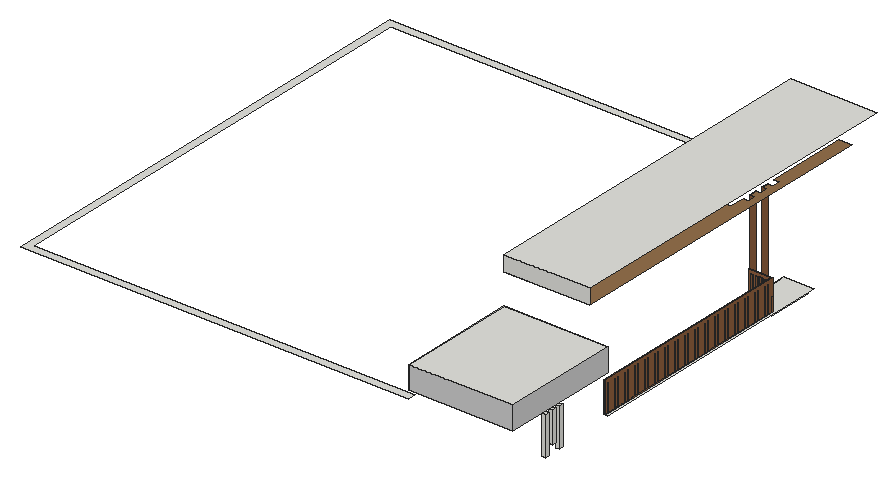
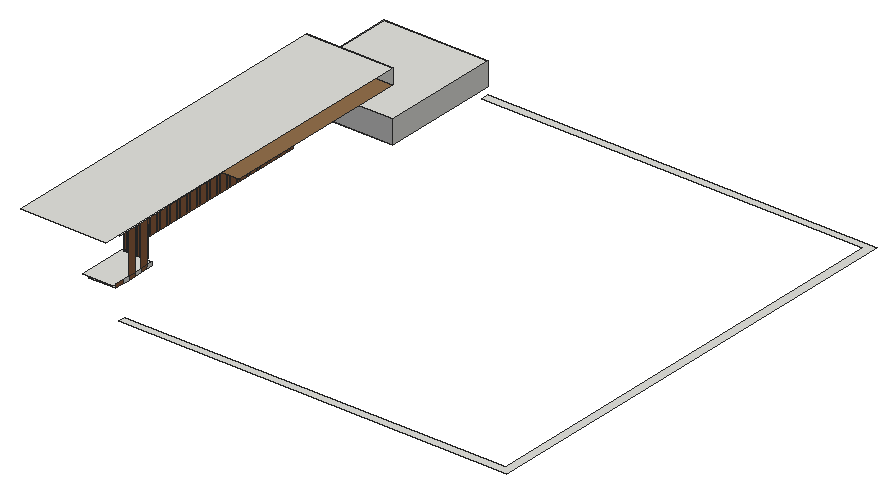
# SketchUp Ruby script. Lengths in inches.
U = 1.inch
M = Sketchup.active_model
def pt(a) = Geom::Point3d.new(a.map { |v| v * U })
def face(e, loops, mat)
  f = e.add_face(loops[0].map { |a| pt(a) })
  loops[1..].each { |l| e.add_face(l.map { |a| pt(a) }).erase! }
  f.material = f.back_material = mat if mat
  f
end
# faces: each face lists its corners as indices into pts; further lists are holes
def faces(e, pts, list, mat = nil) = list.each { |f| face(e, (f[0].is_a?(Array) ? f : [f]).map { |l| l.map { |i| pts[i] } }, mat) }
# xy, xz, yz: faces in a plane at the given z, y or x. An outline is a flat list of corners, or four numbers for a rectangle; further outlines are holes
def ring(l) = l.size == 4 ? [[l[0], l[1]], [l[2], l[1]], [l[2], l[3]], [l[0], l[3]]] : l.each_slice(2).to_a
def flat(e, list, mat, &to3) = list.each { |f| face(e, (f[0].is_a?(Array) ? f : [f]).map { |l| ring(l).map { |u, v| to3.(u, v) } }, mat) }
def xy(e, z, list, mat = nil) = flat(e, list, mat) { |x, y| [x, y, z] }
def xz(e, y, list, mat = nil) = flat(e, list, mat) { |x, z| [x, y, z] }
def yz(e, x, list, mat = nil) = flat(e, list, mat) { |y, z| [x, y, z] }
def lines(e, pts, list) = list.each { |a, b| e.add_line(pt(pts[a]), pt(pts[b])) }
# prism: a flat outline (further loops are holes) pulled along v
def prism(e, loops, v, mat = nil)
  f = face(e, loops, mat); d = Geom::Vector3d.new(v.map { |x| x * U })
  f.pushpull(f.normal.samedirection?(d) ? d.length : -d.length)
end
def box(e, o, s, mat = nil) = prism(e, [[o, [o[0] + s[0], o[1], o[2]], [o[0] + s[0], o[1] + s[1], o[2]], [o[0], o[1] + s[1], o[2]]]], [0, 0, s[2]], mat)
def at(x, y, z, deg = 0) = Geom::Transformation.translation(pt([x, y, z])) * Geom::Transformation.rotation(ORIGIN, Z_AXIS, deg.degrees)
def axes(o, x, y, z) = Geom::Transformation.new([*x, 0, *y, 0, *z, 0, *pt(o).to_a, 1])
def part(name) = M.definitions.add(name)
# library, detail: a bought-in or finely detailed component or shape, given as its bounding box
def library(name, o, s) = part(name).tap { |d| box(d.entities, o, s) }
def detail(e, o, s) = box(e.add_group.entities, o, s)
def put(e, d, t, mat = nil) = e.add_instance(d, t).tap { |i| i.material = mat if mat }
def group(e, t, mat = nil) = e.add_group.tap { |g| g.transformation = t; g.material = mat if mat }.entities
root = M.entities
M.materials.add("M08_Obsidian_Black").color = [30, 30, 30]
M.materials.add("Wood_Floor_01_1K1").color = [146, 111, 76]
M.materials.add("Wood_Veneer_15_1K").color = [142, 95, 62]
M.materials.add("[Cladding_Siding_White]1").color = [207, 207, 207]
xy(root,411,[[360,256,381,291]])
xy(root,414,[[384,28.45,387,31.79],[384,41.79,387,45.12],[382,93,384,93,384,294,360,294,360,256,382,256],[381,93,382,255],[367.6,255,369.4,256],
  [371.2,255,373,256],[374.8,255,376.6,256],[378.4,255,379.7,256],[381,255,382,256]])
xy(root,414,[[365.8,255,367.6,256],[369.4,255,371.2,256],[373,255,374.8,256],[376.6,255,378.4,256],[379.7,255,381,256]],"Wood_Veneer_15_1K")
xy(root,414.5,[[381,187.23,382,187.25],[381,211.625,382,211.68],[381,222.9,382,223],[381,227.875,382,227.98],[381,239.2,382,239.25]])
xy(root,414.5,[[381,94.625,382,96.25],[381,97.875,382,99.5],[381,101.125,382,102.75],[381,104.375,382,105.73],[381,105.73,382,106],
  [381,107.625,382,108.8],[381,108.8,382,109.25],[381,110.875,382,112.5],[381,114.125,382,115.75],[381,117.375,382,119],
  [381,120.625,382,122.02],[381,122.02,382,122.25],[381,123.875,382,125.1],[381,125.1,382,125.5],[381,127.125,382,128.75],
  [381,130.375,382,132],[381,133.625,382,135.25],[381,136.875,382,138.33],[381,138.33,382,138.5],[381,140.125,382,141.4],
  [381,141.4,382,141.75],[381,143.375,382,145],[381,146.625,382,148.25],[381,149.875,382,151.5],[381,153.125,382,154.625],
  [381,154.625,382,154.75],[381,156.375,382,157.7],[381,157.7,382,158],[381,159.625,382,161.25],[381,162.875,382,164.5],
  [381,166.125,382,167.75],[381,169.375,382,170.93],[381,170.93,382,171],[381,172.625,382,174],[381,174,382,174.25],
  [381,175.875,382,177.5],[381,179.125,382,180.75],[381,182.375,382,184],[381,185.625,382,187.23],[381,188.875,382,190.3],
  [381,190.3,382,190.5],[381,192.125,382,193.75],[381,195.375,382,197],[381,198.625,382,200.25],[381,201.875,382,203.5],
  [381,205.125,382,206.6],[381,206.6,382,206.75],[381,208.375,382,210],[381,211.68,382,213.25],[381,214.875,382,216.5],
  [381,218.125,382,219.75],[381,221.375,382,222.9],[381,224.625,382,226.25],[381,227.98,382,229.5],[381,231.125,382,232.75],
  [381,234.375,382,236],[381,237.625,382,239.2],[381,240.875,382,242.5],[381,244.125,382,244.27],[381,244.27,382,245.75],
  [381,247.375,382,249],[381,250.625,382,252.25],[381,253.875,382,255],[381,255,382,255.5]],"Wood_Veneer_15_1K")
xy(root,420,[[384,35.12,387,38.45]])
xy(root,435.5,[[381,117.375,382,117.45]])
xy(root,435.5,[[381,94.625,382,96.25],[381,97.875,382,99.5],[381,101.125,382,102.75],[381,104.375,382,106],[381,107.625,382,109.25],
  [381,110.875,382,112.5],[381,114.125,382,115.75],[381,117.45,382,119],[381,120.625,382,121.52],[381,121.52,382,122.25],
  [381,123.875,382,125.5],[381,127.125,382,128.75],[381,130.375,382,132],[381,133.625,382,133.75],[381,133.75,382,135.25],
  [381,136.875,382,137.83],[381,137.83,382,138.5],[381,140.125,382,141.75],[381,143.375,382,145],[381,146.625,382,148.25],
  [381,149.875,382,150.05],[381,150.05,382,151.5],[381,153.125,382,154.125],[381,154.125,382,154.75],[381,156.375,382,158],
  [381,159.625,382,161.25],[381,162.875,382,164.5],[381,166.125,382,166.35],[381,166.35,382,167.75],[381,169.375,382,170.43],
  [381,170.43,382,171],[381,172.625,382,174.25],[381,175.875,382,177.5],[381,179.125,382,180.75],[381,182.375,382,182.65],
  [381,182.65,382,184],[381,185.625,382,186.73],[381,186.73,382,187.25],[381,188.875,382,190.5],[381,192.125,382,193.75],
  [381,195.375,382,197],[381,198.625,382,198.95],[381,198.95,382,200.25],[381,201.875,382,203.03],[381,203.03,382,203.5],
  [381,205.125,382,206.75],[381,208.375,382,210],[381,211.625,382,213.25],[381,214.875,382,215.25],[381,215.25,382,216.5],
  [381,218.125,382,219.33],[381,219.33,382,219.75],[381,221.375,382,223],[381,224.625,382,226.25],[381,227.875,382,229.5],
  [381,231.125,382,231.55],[381,231.55,382,232.75],[381,234.375,382,235.625],[381,235.625,382,236],[381,237.625,382,239.25],
  [381,240.875,382,242.5],[381,244.125,382,245.75],[381,247.375,382,247.85],[381,247.85,382,249],[381,250.625,382,251.92],
  [381,251.92,382,252.25],[381,253.875,382,255.5],[365.8,255,367.6,256],[369.4,255,371.2,256],[373,255,374.8,256],
  [376.6,255,378.4,256],[379.7,255,381,256]],"Wood_Veneer_15_1K")
xy(root,438,[[0,0,303,0,303,6,6,6,6,354,303,354,303,360,0,360]])
xy(root,438,[[381,93,382,93,382,256,364,256,364,255,381,255]],"Wood_Veneer_15_1K")
xy(root,444,[[303,0,384,9],[303,9,309,93],[309,9,375,87],[375,9,384,93],[384,28.45,387,31.79],
  [384,35.12,387,38.45],[384,41.79,387,45.12],[309,87,375,93]])
xy(root,462,[[303,0,384,93]])
xy(root,480,[[354,294,360,336]],"M08_Obsidian_Black")
xy(root,486,[[303,93,303,243,360,243,360,255,364,255,364,261,360,261,360,267,364,267,364,273,360,273,360,279,364,279,364,285,360,285,360,348,370,348,370,93]],"Wood_Floor_01_1K1")
xy(root,492,[[309,249,351,351]])
xy(root,498,[[303,93,370,372]])
xz(root,0,[[303,444,384,462]],"[Cladding_Siding_White]1")
xz(root,28.45,[[384,414,387,444]])
xz(root,31.79,[[384,414,387,444]])
xz(root,35.12,[[384,420,387,444]])
xz(root,38.45,[[384,420,387,444]])
xz(root,41.79,[[384,414,387,444]])
xz(root,45.12,[[384,414,387,444]])
xz(root,93,[[303,486,370,498]])
xz(root,93,[[381,414,382,438],[303,444,384,462]],"[Cladding_Siding_White]1")
xz(root,94.625,[[381,414.5,382,435.5]],"Wood_Veneer_15_1K")
xz(root,96.25,[[381,414.5,382,435.5]],"Wood_Veneer_15_1K")
xz(root,97.875,[[381,414.5,382,435.5]],"Wood_Veneer_15_1K")
xz(root,99.5,[[381,414.5,382,435.5]],"Wood_Veneer_15_1K")
xz(root,101.125,[[381,414.5,382,435.5]],"Wood_Veneer_15_1K")
xz(root,102.75,[[381,414.5,382,435.5]],"Wood_Veneer_15_1K")
xz(root,104.375,[[381,414.5,382,435.5]],"Wood_Veneer_15_1K")
xz(root,106,[[381,414.5,382,435.5]],"Wood_Veneer_15_1K")
xz(root,107.625,[[381,414.5,382,435.5]],"Wood_Veneer_15_1K")
xz(root,109.25,[[381,414.5,382,435.5]],"Wood_Veneer_15_1K")
xz(root,110.875,[[381,414.5,382,435.5]],"Wood_Veneer_15_1K")
xz(root,112.5,[[381,414.5,382,435.5]],"Wood_Veneer_15_1K")
xz(root,114.125,[[381,414.5,382,435.5]],"Wood_Veneer_15_1K")
xz(root,115.75,[[381,414.5,382,435.5]],"Wood_Veneer_15_1K")
xz(root,117.375,[[381,414.5,382,435.5]],"Wood_Veneer_15_1K")
xz(root,119,[[381,414.5,382,435.5]],"Wood_Veneer_15_1K")
xz(root,120.625,[[381,414.5,382,435.5]],"Wood_Veneer_15_1K")
xz(root,122.25,[[381,414.5,382,435.5]],"Wood_Veneer_15_1K")
xz(root,123.875,[[381,414.5,382,435.5]],"Wood_Veneer_15_1K")
xz(root,125.5,[[381,414.5,382,435.5]],"Wood_Veneer_15_1K")
xz(root,127.125,[[381,414.5,382,435.5]],"Wood_Veneer_15_1K")
xz(root,128.75,[[381,414.5,382,435.5]],"Wood_Veneer_15_1K")
xz(root,130.375,[[381,414.5,382,435.5]],"Wood_Veneer_15_1K")
xz(root,132,[[381,414.5,382,435.5]],"Wood_Veneer_15_1K")
xz(root,133.625,[[381,414.5,382,435.5]],"Wood_Veneer_15_1K")
xz(root,135.25,[[381,414.5,382,435.5]],"Wood_Veneer_15_1K")
xz(root,136.875,[[381,414.5,382,435.5]],"Wood_Veneer_15_1K")
xz(root,138.5,[[381,414.5,382,435.5]],"Wood_Veneer_15_1K")
xz(root,140.125,[[381,414.5,382,435.5]],"Wood_Veneer_15_1K")
xz(root,141.75,[[381,414.5,382,435.5]],"Wood_Veneer_15_1K")
xz(root,143.375,[[381,414.5,382,435.5]],"Wood_Veneer_15_1K")
xz(root,145,[[381,414.5,382,435.5]],"Wood_Veneer_15_1K")
xz(root,146.625,[[381,414.5,382,435.5]],"Wood_Veneer_15_1K")
xz(root,148.25,[[381,414.5,382,435.5]],"Wood_Veneer_15_1K")
xz(root,149.875,[[381,414.5,382,435.5]],"Wood_Veneer_15_1K")
xz(root,151.5,[[381,414.5,382,435.5]],"Wood_Veneer_15_1K")
xz(root,153.125,[[381,414.5,382,435.5]],"Wood_Veneer_15_1K")
xz(root,154.75,[[381,414.5,382,435.5]],"Wood_Veneer_15_1K")
xz(root,156.375,[[381,414.5,382,435.5]],"Wood_Veneer_15_1K")
xz(root,158,[[381,414.5,382,435.5]],"Wood_Veneer_15_1K")
xz(root,159.625,[[381,414.5,382,435.5]],"Wood_Veneer_15_1K")
xz(root,161.25,[[381,414.5,382,435.5]],"Wood_Veneer_15_1K")
xz(root,162.875,[[381,414.5,382,435.5]],"Wood_Veneer_15_1K")
xz(root,164.5,[[381,414.5,382,435.5]],"Wood_Veneer_15_1K")
xz(root,166.125,[[381,414.5,382,435.5]],"Wood_Veneer_15_1K")
xz(root,167.75,[[381,414.5,382,435.5]],"Wood_Veneer_15_1K")
xz(root,169.375,[[381,414.5,382,435.5]],"Wood_Veneer_15_1K")
xz(root,171,[[381,414.5,382,435.5]],"Wood_Veneer_15_1K")
xz(root,172.625,[[381,414.5,382,435.5]],"Wood_Veneer_15_1K")
xz(root,174.25,[[381,414.5,382,435.5]],"Wood_Veneer_15_1K")
xz(root,175.875,[[381,414.5,382,435.5]],"Wood_Veneer_15_1K")
xz(root,177.5,[[381,414.5,382,435.5]],"Wood_Veneer_15_1K")
xz(root,179.125,[[381,414.5,382,435.5]],"Wood_Veneer_15_1K")
xz(root,180.75,[[381,414.5,382,435.5]],"Wood_Veneer_15_1K")
xz(root,182.375,[[381,414.5,382,435.5]],"Wood_Veneer_15_1K")
xz(root,184,[[381,414.5,382,435.5]],"Wood_Veneer_15_1K")
xz(root,185.625,[[381,414.5,382,435.5]],"Wood_Veneer_15_1K")
xz(root,187.25,[[381,414.5,382,435.5]],"Wood_Veneer_15_1K")
xz(root,188.875,[[381,414.5,382,435.5]],"Wood_Veneer_15_1K")
xz(root,190.5,[[381,414.5,382,435.5]],"Wood_Veneer_15_1K")
xz(root,192.125,[[381,414.5,382,435.5]],"Wood_Veneer_15_1K")
xz(root,193.75,[[381,414.5,382,435.5]],"Wood_Veneer_15_1K")
xz(root,195.375,[[381,414.5,382,435.5]],"Wood_Veneer_15_1K")
xz(root,197,[[381,414.5,382,435.5]],"Wood_Veneer_15_1K")
xz(root,198.625,[[381,414.5,382,435.5]],"Wood_Veneer_15_1K")
xz(root,200.25,[[381,414.5,382,435.5]],"Wood_Veneer_15_1K")
xz(root,201.875,[[381,414.5,382,435.5]],"Wood_Veneer_15_1K")
xz(root,203.5,[[381,414.5,382,435.5]],"Wood_Veneer_15_1K")
xz(root,205.125,[[381,414.5,382,435.5]],"Wood_Veneer_15_1K")
xz(root,206.75,[[381,414.5,382,435.5]],"Wood_Veneer_15_1K")
xz(root,208.375,[[381,414.5,382,435.5]],"Wood_Veneer_15_1K")
xz(root,210,[[381,414.5,382,435.5]],"Wood_Veneer_15_1K")
xz(root,211.625,[[381,414.5,382,435.5]],"Wood_Veneer_15_1K")
xz(root,213.25,[[381,414.5,382,435.5]],"Wood_Veneer_15_1K")
xz(root,214.875,[[381,414.5,382,435.5]],"Wood_Veneer_15_1K")
xz(root,216.5,[[381,414.5,382,435.5]],"Wood_Veneer_15_1K")
xz(root,218.125,[[381,414.5,382,435.5]],"Wood_Veneer_15_1K")
xz(root,219.75,[[381,414.5,382,435.5]],"Wood_Veneer_15_1K")
xz(root,221.375,[[381,414.5,382,435.5]],"Wood_Veneer_15_1K")
xz(root,223,[[381,414.5,382,435.5]],"Wood_Veneer_15_1K")
xz(root,224.625,[[381,414.5,382,435.5]],"Wood_Veneer_15_1K")
xz(root,226.25,[[381,414.5,382,435.5]],"Wood_Veneer_15_1K")
xz(root,227.875,[[381,414.5,382,435.5]],"Wood_Veneer_15_1K")
xz(root,229.5,[[381,414.5,382,435.5]],"Wood_Veneer_15_1K")
xz(root,231.125,[[381,414.5,382,435.5]],"Wood_Veneer_15_1K")
xz(root,232.75,[[381,414.5,382,435.5]],"Wood_Veneer_15_1K")
xz(root,234.375,[[381,414.5,382,435.5]],"Wood_Veneer_15_1K")
xz(root,236,[[381,414.5,382,435.5]],"Wood_Veneer_15_1K")
xz(root,237.625,[[381,414.5,382,435.5]],"Wood_Veneer_15_1K")
xz(root,239.25,[[381,414.5,382,435.5]],"Wood_Veneer_15_1K")
xz(root,240.875,[[381,414.5,382,435.5]],"Wood_Veneer_15_1K")
xz(root,242.5,[[381,414.5,382,435.5]],"Wood_Veneer_15_1K")
xz(root,244.125,[[381,414.5,382,435.5]],"Wood_Veneer_15_1K")
xz(root,245.75,[[381,414.5,382,435.5]],"Wood_Veneer_15_1K")
xz(root,247.375,[[381,414.5,382,435.5]],"Wood_Veneer_15_1K")
xz(root,249,[[381,414.5,382,435.5]],"Wood_Veneer_15_1K")
xz(root,250.625,[[381,414.5,382,435.5]],"Wood_Veneer_15_1K")
xz(root,252.25,[[381,414.5,382,435.5]],"Wood_Veneer_15_1K")
xz(root,253.875,[[381,414.5,382,435.5]],"Wood_Veneer_15_1K")
xz(root,255,[[364,414,365.8,414,365.8,435.5,367.6,435.5,367.6,414,369.4,414,369.4,435.5,371.2,435.5,371.2,414,373,414,373,435.5,374.8,435.5,374.8,414,376.6,414,376.6,435.5,378.4,435.5,378.4,414,379.7,414,379.7,435.5,381,435.5,381,438,364,438]],"Wood_Veneer_15_1K")
xz(root,255.5,[[381,414.5,382,435.5]],"Wood_Veneer_15_1K")
xz(root,256,[[360,411,364,414],[364,411,381,414]])
xz(root,256,[[364,414,364,438,382,438,382,414,381,414,381,435.5,379.7,435.5,379.7,414,378.4,414,378.4,435.5,376.6,435.5,376.6,414,374.8,414,374.8,435.5,373,435.5,373,414,371.2,414,371.2,435.5,369.4,435.5,369.4,414,367.6,414,367.6,435.5,365.8,435.5,365.8,414]],"Wood_Veneer_15_1K")
yz(root,303,[[0,444,93,462]])
yz(root,360,[[256,411,261,414],[267,411,273,414],[279,411,285,414]])
yz(root,360,[[261,411,267,414],[273,411,279,414],[285,411,291,414],[261,414,267,486],[273,414,279,486]],"Wood_Veneer_15_1K")
yz(root,365.8,[[255,414,256,435.5]],"Wood_Veneer_15_1K")
yz(root,367.6,[[255,414,256,435.5]],"Wood_Veneer_15_1K")
yz(root,369.4,[[255,414,256,435.5]],"Wood_Veneer_15_1K")
yz(root,371.2,[[255,414,256,435.5]],"Wood_Veneer_15_1K")
yz(root,373,[[255,414,256,435.5]],"Wood_Veneer_15_1K")
yz(root,374.8,[[255,414,256,435.5]],"Wood_Veneer_15_1K")
yz(root,376.6,[[255,414,256,435.5]],"Wood_Veneer_15_1K")
yz(root,378.4,[[255,414,256,435.5]],"Wood_Veneer_15_1K")
yz(root,379.7,[[255,414,256,435.5]],"Wood_Veneer_15_1K")
yz(root,381,[[[93,414,93,438,255,438,255,435.5,253.875,435.5,253.875,414.5,255,414.5,255,414],[250.625,414.5,252.25,435.5],[247.375,414.5,249,435.5],[240.875,414.5,242.5,435.5],[234.375,414.5,236,435.5],[231.125,414.5,232.75,435.5],[224.625,414.5,226.25,435.5],[218.125,414.5,219.75,435.5],[214.875,414.5,216.5,435.5],[208.375,414.5,210,435.5],[201.875,414.5,203.5,435.5],[198.625,414.5,200.25,435.5],[192.125,414.5,193.75,435.5],[182.375,414.5,184,435.5],[179.125,414.5,180.75,435.5],[175.875,414.5,177.5,435.5],[166.125,414.5,167.75,435.5],[162.875,414.5,164.5,435.5],[159.625,414.5,161.25,435.5],[149.875,414.5,151.5,435.5],[146.625,414.5,148.25,435.5],[143.375,414.5,145,435.5],[133.625,414.5,135.25,435.5],[130.375,414.5,132,435.5],[127.125,414.5,128.75,435.5],[117.375,414.5,119,435.5],[114.125,414.5,115.75,435.5],[110.875,414.5,112.5,435.5],[101.125,414.5,102.75,435.5],[97.875,414.5,99.5,435.5],[94.625,414.5,96.25,435.5],[188.875,414.5,190.5,435.5],[136.875,414.5,138.5,435.5],[107.625,414.5,109.25,435.5],[104.375,414.5,106,435.5],[244.125,414.5,245.75,435.5],[237.625,414.5,239.25,435.5],[227.875,414.5,229.5,435.5],[221.375,414.5,223,435.5],[211.625,414.5,213.25,435.5],[205.125,414.5,206.75,435.5],[195.375,414.5,197,435.5],[185.625,414.5,187.25,435.5],[172.625,414.5,174.25,435.5],[169.375,414.5,171,435.5],[156.375,414.5,158,435.5],[153.125,414.5,154.75,435.5],[140.125,414.5,141.75,435.5],[123.875,414.5,125.5,435.5],[120.625,414.5,122.25,435.5]],[255,414,255,414.5,255.5,414.5,255.5,435.5,256,435.5,256,414]],"Wood_Veneer_15_1K")
yz(root,382,[[93,414,256,414,256,425.5,255.5,425.5,255.5,414.5,93,414.5],[93,414.5,94.625,414.5,94.625,435.5,96.25,435.5,96.25,414.5,97.875,414.5,97.875,435.5,99.5,435.5,99.5,414.5,101.125,414.5,101.125,435.5,102.75,435.5,102.75,414.5,104.375,414.5,104.375,435.5,106,435.5,106,414.5,107.625,414.5,107.625,435.5,109.25,435.5,109.25,414.5,110.875,414.5,110.875,435.5,112.5,435.5,112.5,414.5,114.125,414.5,114.125,435.5,115.75,435.5,115.75,414.5,117.375,414.5,117.375,435.5,119,435.5,119,414.5,120.625,414.5,120.625,435.5,122.25,435.5,122.25,414.5,123.875,414.5,123.875,435.5,125.5,435.5,125.5,414.5,127.125,414.5,127.125,435.5,128.75,435.5,128.75,414.5,130.375,414.5,130.375,435.5,132,435.5,132,414.5,133.625,414.5,133.625,435.5,135.25,435.5,135.25,414.5,136.875,414.5,136.875,435.5,138.5,435.5,138.5,414.5,140.125,414.5,140.125,435.5,141.75,435.5,141.75,414.5,143.375,414.5,143.375,435.5,145,435.5,145,414.5,146.625,414.5,146.625,435.5,148.25,435.5,148.25,414.5,149.875,414.5,149.875,435.5,151.5,435.5,151.5,414.5,153.125,414.5,153.125,435.5,154.75,435.5,154.75,414.5,156.375,414.5,156.375,435.5,158,435.5,158,414.5,159.625,414.5,159.625,435.5,161.25,435.5,161.25,414.5,162.875,414.5,162.875,435.5,164.5,435.5,164.5,414.5,166.125,414.5,166.125,435.5,167.75,435.5,167.75,414.5,169.375,414.5,169.375,435.5,171,435.5,171,414.5,172.625,414.5,172.625,435.5,174.25,435.5,174.25,414.5,175.875,414.5,175.875,435.5,177.5,435.5,177.5,414.5,179.125,414.5,179.125,435.5,180.75,435.5,180.75,414.5,182.375,414.5,182.375,435.5,184,435.5,184,414.5,185.625,414.5,185.625,435.5,187.25,435.5,187.25,414.5,188.875,414.5,188.875,435.5,190.5,435.5,190.5,414.5,192.125,414.5,192.125,435.5,193.75,435.5,193.75,414.5,195.375,414.5,195.375,435.5,197,435.5,197,414.5,198.625,414.5,198.625,435.5,200.25,435.5,200.25,414.5,201.875,414.5,201.875,435.5,203.5,435.5,203.5,414.5,205.125,414.5,205.125,435.5,206.75,435.5,206.75,414.5,208.375,414.5,208.375,435.5,210,435.5,210,414.5,211.625,414.5,211.625,435.5,213.25,435.5,213.25,414.5,214.875,414.5,214.875,435.5,216.5,435.5,216.5,414.5,218.125,414.5,218.125,435.5,219.75,435.5,219.75,414.5,221.375,414.5,221.375,435.5,223,435.5,223,414.5,224.625,414.5,224.625,435.5,226.25,435.5,226.25,414.5,227.875,414.5,227.875,435.5,229.5,435.5,229.5,414.5,231.125,414.5,231.125,435.5,232.75,435.5,232.75,414.5,234.375,414.5,234.375,435.5,236,435.5,236,414.5,237.625,414.5,237.625,435.5,239.25,435.5,239.25,414.5,240.875,414.5,240.875,435.5,242.5,435.5,242.5,414.5,244.125,414.5,244.125,435.5,245.75,435.5,245.75,414.5,247.375,414.5,247.375,435.5,249,435.5,249,414.5,250.625,414.5,250.625,435.5,252.25,435.5,252.25,414.5,253.875,414.5,253.875,435.5,255.5,435.5,255.5,425.5,256,425.5,256,438,93,438]],"Wood_Veneer_15_1K")
yz(root,384,[[0,444,93,462]],"[Cladding_Siding_White]1")
yz(root,387,[[28.45,414,31.79,444],[41.79,414,45.12,444],[35.12,420,38.45,444]])
p = [[351,351,492],[351,351,498],[309,351,492],[309,351,498],[309,249,492],[309,249,498],
  [351,249,492],[351,249,498]]
lines(root,p,[[0,1],[2,3],[4,5],[6,7]])
